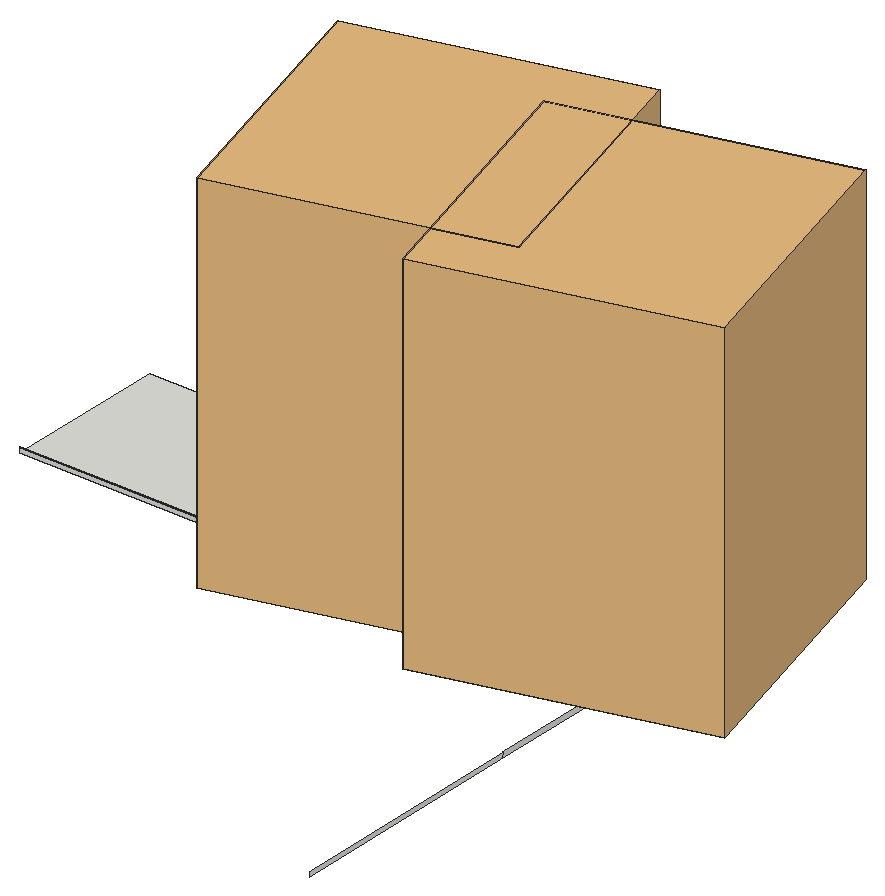
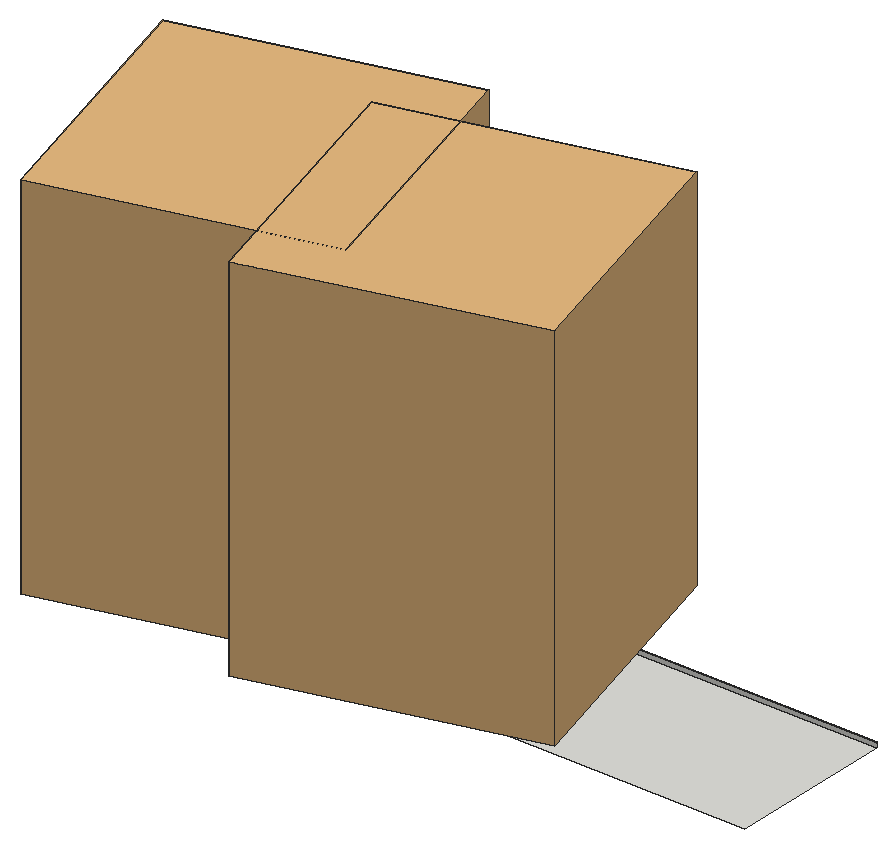
# SketchUp Ruby script. Lengths in inches.
U = 1.inch
M = Sketchup.active_model
def pt(a) = Geom::Point3d.new(a.map { |v| v * U })
def face(e, loops, mat)
  f = e.add_face(loops[0].map { |a| pt(a) })
  loops[1..].each { |l| e.add_face(l.map { |a| pt(a) }).erase! }
  f.material = f.back_material = mat if mat
  f
end
# faces: each face lists its corners as indices into pts; further lists are holes
def faces(e, pts, list, mat = nil) = list.each { |f| face(e, (f[0].is_a?(Array) ? f : [f]).map { |l| l.map { |i| pts[i] } }, mat) }
# xy, xz, yz: faces in a plane at the given z, y or x. An outline is a flat list of corners, or four numbers for a rectangle; further outlines are holes
def ring(l) = l.size == 4 ? [[l[0], l[1]], [l[2], l[1]], [l[2], l[3]], [l[0], l[3]]] : l.each_slice(2).to_a
def flat(e, list, mat, &to3) = list.each { |f| face(e, (f[0].is_a?(Array) ? f : [f]).map { |l| ring(l).map { |u, v| to3.(u, v) } }, mat) }
def xy(e, z, list, mat = nil) = flat(e, list, mat) { |x, y| [x, y, z] }
def xz(e, y, list, mat = nil) = flat(e, list, mat) { |x, z| [x, y, z] }
def yz(e, x, list, mat = nil) = flat(e, list, mat) { |y, z| [x, y, z] }
def lines(e, pts, list) = list.each { |a, b| e.add_line(pt(pts[a]), pt(pts[b])) }
# prism: a flat outline (further loops are holes) pulled along v
def prism(e, loops, v, mat = nil)
  f = face(e, loops, mat); d = Geom::Vector3d.new(v.map { |x| x * U })
  f.pushpull(f.normal.samedirection?(d) ? d.length : -d.length)
end
def box(e, o, s, mat = nil) = prism(e, [[o, [o[0] + s[0], o[1], o[2]], [o[0] + s[0], o[1] + s[1], o[2]], [o[0], o[1] + s[1], o[2]]]], [0, 0, s[2]], mat)
def at(x, y, z, deg = 0) = Geom::Transformation.translation(pt([x, y, z])) * Geom::Transformation.rotation(ORIGIN, Z_AXIS, deg.degrees)
def axes(o, x, y, z) = Geom::Transformation.new([*x, 0, *y, 0, *z, 0, *pt(o).to_a, 1])
def part(name) = M.definitions.add(name)
# library, detail: a bought-in or finely detailed component or shape, given as its bounding box
def library(name, o, s) = part(name).tap { |d| box(d.entities, o, s) }
def detail(e, o, s) = box(e.add_group.entities, o, s)
def put(e, d, t, mat = nil) = e.add_instance(d, t).tap { |i| i.material = mat if mat }
def group(e, t, mat = nil) = e.add_group.tap { |g| g.transformation = t; g.material = mat if mat }.entities
root = M.entities
M.materials.add("Material82").color = [68, 110, 58]
M.materials.add("Material83").color = [48, 90, 38]
M.materials.add("Material84").color = [68, 110, 48]
M.materials.add("Material85").color = [48, 90, 48]
M.materials.add("Material86").color = [58, 110, 58]
M.materials.add("Material87").color = [58, 90, 38]
M.materials.add("Material88").color = [68, 100, 58]
M.materials.add("Material89").color = [48, 100, 38]
c1 = part("grass00")
p = [[-0.6875,0.15,0],[-0.56,0.08,5.52],[-0.04,0.03,2.76],[0.48,-0.02,0],[0.35,-0.02,5.52],[-0.1,-0.14,5.52],
  [-0.12,0.65,8.37],[-0.42,0.65,8.37]]
faces(c1.entities,p,[[0,1,2,3],[3,2,4],[1,5,2],[5,4,2],[1,6,5],[4,5,6],[7,6,1]])
c2 = part("Group16\#1")
put(c2.entities,c1,axes([1.44,-0.61,-0.01],[0.05352,0.12609,0],[-0.10704,0.04543,0.07239],[0.06664,-0.02828,0.11628]),"Material85")
put(c2.entities,c1,axes([0.76,-0.15,-0.01],[0.04676,0.24062,0],[-0.23162,0.04501,0.06642],[0.0652,-0.01267,0.23595]),"Material82")
put(c2.entities,c1,axes([0.79,0.01,-0.01],[-0.00606,0.34651,0],[-0.34381,-0.00602,0.0432],[0.04319,0.00076,0.34386]))
put(c2.entities,c1,axes([1,0.23,-0.01],[-0.07192,0.31144,0],[-0.28722,-0.06632,0.1236],[0.12043,0.02781,0.29478]),"Material84")
put(c2.entities,c1,axes([1.66,0.77,-0.01],[-0.13828,0.29651,0],[-0.21551,-0.1005,0.22471],[0.20365,0.09498,0.23779]),"Material89")
put(c2.entities,c1,axes([0.6875,0.52,-0.01],[-0.18126,0.24051,0],[-0.22746,-0.17142,0.09788],[0.07817,0.05891,0.28481]),"Material84")
put(c2.entities,c1,axes([0.68,0.78,-0.01],[-0.215,0.18688,0],[-0.12385,-0.14248,0.21334],[0.13995,0.16101,0.18878]),"Material82")
put(c2.entities,c1,axes([0.56,1,-0.01],[-0.13756,0.07624,0],[-0.06159,-0.11112,0.0927],[0.04494,0.08108,0.12705]),"Material84")
put(c2.entities,c1,axes([0.2,0.64,-0.01],[-0.23729,0.07254,0],[-0.05711,-0.18681,0.153],[0.04473,0.14632,0.19535]),"Material89")
put(c2.entities,c1,axes([0.0625,0.72,-0.01],[-0.28874,0.02525,0],[-0.02179,-0.24916,0.14647],[0.01276,0.14591,0.25012]),"Material82")
put(c2.entities,c1,axes([-0.08,0.62,-0.01],[-0.34089,-0.04187,0],[0.03255,-0.26504,0.216],[-0.02633,0.21439,0.26703]),"Material89")
put(c2.entities,c1,axes([-0.34,0.98,-0.01],[-0.14314,-0.0493,0],[0.04397,-0.12769,0.06843],[-0.02228,0.0647,0.13505]),"Material89")
put(c2.entities,c1,axes([-0.87,1.45,-0.01],[-0.23488,-0.14114,0],[0.13761,-0.22901,0.06087],[-0.03135,0.05217,0.26717]))
put(c2.entities,c1,axes([-0.72,0.77,-0.01],[-0.14208,-0.13251,0],[0.07209,-0.0773,0.16301],[-0.11118,0.11922,0.1057]),"Material89")
put(c2.entities,c1,axes([-0.62,0.43,-0.01],[-0.14845,-0.21203,0],[0.18654,-0.13061,0.12304],[-0.10079,0.07057,0.22772]),"Material82")
put(c2.entities,c1,axes([-0.68,0.29,-0.01],[-0.13639,-0.32136,0],[0.31723,-0.13464,0.05579],[-0.05136,0.0218,0.34462]),"Material83")
put(c2.entities,c1,axes([-0.64,0.125,-0.01],[-0.0458,-0.23569,0],[0.22124,-0.043,0.08276],[-0.08124,0.01579,0.22538]),"Material86")
put(c2.entities,c1,axes([-1.6,-0.03,-0.01],[0.00576,-0.32897,0],[0.27526,0.00482,0.18018],[-0.18015,-0.00315,0.2753]),"Material84")
put(c2.entities,c1,axes([-1.36,-0.31,-0.01],[0.05718,-0.24765,0],[0.18172,0.04196,0.17267],[-0.16825,-0.03885,0.1865]),"Material89")
put(c2.entities,c1,axes([-1.54,-0.72,-0.01],[0.06537,-0.14017,0],[0.13555,0.06321,0.03939],[-0.0357,-0.01665,0.14956]))
put(c2.entities,c1,axes([-1.19,-0.9,-0.01],[0.09597,-0.12735,0],[0.11214,0.08451,0.07557],[-0.06035,-0.04548,0.14042]),"Material88")
put(c2.entities,c1,axes([-0.47,-0.54,-0.01],[0.11588,-0.10072,0],[0.0618,0.0711,0.12124],[-0.07953,-0.0915,0.0942]))
put(c2.entities,c1,axes([-0.47,-0.84,-0.01],[0.11927,-0.0661,0],[0.06603,0.11913,0.00646],[-0.00313,-0.00565,0.13621]),"Material84")
put(c2.entities,c1,axes([-0.38,-1.24,-0.01],[0.28037,-0.08571,0],[0.0618,0.20215,0.20315],[-0.05939,-0.19428,0.21139]),"Material88")
put(c2.entities,c1,axes([-0.06,-0.66,-0.01],[0.22719,-0.01987,0],[0.01247,0.14255,0.17758],[-0.01547,-0.17691,0.1431]),"Material87")
put(c2.entities,c1,axes([0.11,-0.89,-0.01],[0.14882,0.01828,0],[-0.01058,0.08611,0.12229],[0.01491,-0.12138,0.08676]),"Material85")
put(c2.entities,c1,axes([0.25,-0.72,-0.01],[0.20481,0.07053,0],[-0.06206,0.18022,0.10291],[0.03351,-0.0973,0.1906]),"Material85")
put(c2.entities,c1,axes([0.85,-1.42,-0.01],[0.16481,0.09904,0],[-0.09472,0.15762,0.05616],[0.02893,-0.04814,0.18389]),"Material84")
put(c2.entities,c1,axes([1.01,-1.09,-0.01],[0.21858,0.20385,0],[-0.17495,0.1876,0.15339],[0.10462,-0.11218,0.25652]),"Material89")
put(c2.entities,c1,axes([1.01,-0.71,-0.01],[0.08733,0.12473,0],[-0.06445,0.04512,0.13037],[0.1068,-0.07477,0.07867]),"Material85")
c3 = part("Group15\#1")
put(c3.entities,c2,at(0,0,0))
c4 = part("3darcstudiotree_grass00\#1")
put(c4.entities,c3,at(0,0,0))
c5 = library("Palm tree",[-4.09,-4.52,0],[193.52,193.51,258.93])
c6 = part("Palm+Tree")
put(c6.entities,c5,at(25.51,-21.81,0,15))
c7 = library("Group\#612",[0,0,0],[32.91,53.52,103.45])
xy(root,-42.1875,[[1674.99,273.41,2096.97,387.84]])
xz(root,273.41,[[1674.99,-42.1875,2096.97,-42.1875,2096.97,-38.61,1897.28,-38.61,1897.28,-39.125,1674.99,-39.125],[1674.99,-38.61,2096.97,-38.1875]])
yz(root,2096.97,[[1.59,-42.1875,172.28,-39.1875],[172.28,-42.1875,273.41,-38.61],[273.41,-42.1875,387.84,-34.17]])
put(root,c4,axes([1856.99,323.88,-34.17],[-2.27595,1.46975,0],[-3.85308,-0.92798,-0.0342],[-0.14118,-0.034,1.63693]))
put(root,c4,axes([1856.66,307.49,-34.17],[3.38368,1.04745,0],[-2.27938,1.14521,-0.02005],[-0.08327,0.04184,1.86077]))
put(root,c4,axes([1858.71,335.1875,-34.17],[0.01113,-1.45353,0],[4.54919,0.00542,-0.03692],[0.17089,0.0002,1.57831]))
put(root,c4,axes([1859.04,313.29,-34.17],[-1.2969,-1.20265,0],[3.80092,-0.63749,-0.01791],[0.10113,-0.01696,1.89984]))
put(root,c4,axes([1859.15,291.65,-34.17],[0.25593,-1.38573,0],[3.33259,0.09573,-0.00937],[0.07232,0.00208,1.93766]))
put(root,c4,axes([1859.03,287.07,-34.17],[-3.13946,0.49629,0],[-1.50487,-1.48058,-0.04281],[-0.09532,-0.09378,1.81418]))
put(root,c4,axes([1858.93,329.8125,-34.17],[3.11316,-1.08854,0],[2.76667,1.23063,-0.03392],[0.0954,0.04244,1.32537]))
put(root,c4,axes([1860.03,298.21,-34.17],[-3.90762,0.14516,0],[-0.37668,-1.57704,-0.0202],[-0.01231,-0.05153,1.95637]))
put(root,c4,axes([1860.17,339.86,-34.17],[-1.14276,-1.73672,0],[3.49011,-0.35717,-0.03225],[0.18285,-0.01871,1.58326]))
put(root,c4,axes([1858.89,282.42,-34.17],[3.63772,-0.04618,0],[0.1059,1.29755,-0.04101],[0.00733,0.08987,1.37186]))
put(root,c4,axes([1858.96,337.85,-34.17],[0.13497,1.53866,0],[-3.75353,0.05121,-0.02489],[-0.17047,0.00233,1.9295]))
put(root,c4,axes([1859.52,333.37,-34.17],[-2.50392,0.92561,0],[-3.00944,-1.26617,-0.02311],[-0.06646,-0.02796,1.38694]))
put(root,c4,axes([1860.67,326.64,-34.17],[-4.13167,0.24366,0],[-0.69238,-1.82599,-0.06496],[-0.05165,-0.1362,1.88637]))
put(root,c4,axes([1859.86,309.54,-34.17],[-1.70819,1.11812,0],[-3.96876,-0.943,-0.04504],[-0.21667,-0.05148,1.9506]))
put(root,c4,axes([1860.05,318.65,-34.17],[3.79912,-1.05543,0],[2.19489,1.22878,-0.03692],[0.13668,0.07652,1.83631]))
put(root,c4,axes([1859.92,284.9,-34.17],[3.28657,0.21022,0],[-0.53923,1.31117,-0.01255],[-0.01302,0.03166,1.63564]))
put(root,c4,axes([1860.52,324.84,-34.17],[-2.37455,1.29783,0],[-2.73236,-0.77752,-0.00844],[-0.03827,-0.01089,1.41311]))
put(root,c4,axes([1859.85,315.9,-34.17],[2.3712,1.21069,0],[-3.58151,1.09097,-0.04605],[-0.15475,0.04714,1.44046]))
put(root,c4,axes([1861.08,301.02,-34.17],[1.66455,-1.14728,0],[3.31311,0.74761,-0.04415],[0.26641,0.06012,1.98924]))
put(root,c4,axes([1862.18,331.24,-34.17],[-0.63027,-1.58552,0],[4.65732,-0.28794,-0.06318],[0.24644,-0.01524,1.39517]))
put(root,c4,axes([1860.64,302.46,-34.17],[2.52471,1.58546,0],[-3.52346,0.87265,-0.052],[-0.25077,0.06211,1.7759]))
put(root,c4,axes([1861.42,323.25,-34.17],[3.33412,-1.28398,0],[2.96352,1.19685,-0.04175],[0.14903,0.06019,1.62422]))
put(root,c4,axes([1860.82,319.77,-34.17],[3.98735,0.11869,0],[-0.3473,1.81468,-0.00004],[-0.00002,0.00009,1.93334]))
put(root,c4,axes([1862.46,294.22,-34.17],[-2.08457,-1.53905,0],[3.84719,-0.81044,-0.05822],[0.30315,-0.06386,1.92982]))
put(root,c4,axes([1861.59,311.12,-34.17],[0.24653,1.78059,0],[-4.18646,0.09015,-0.05861],[-0.36644,0.00789,1.96776]))
put(root,c4,axes([1861.1,305.77,-34.17],[4.09909,0.70116,0],[-1.55013,1.40946,-0.01845],[-0.03388,0.03081,1.34771]))
put(root,c4,axes([1861.13,281.39,-34.17],[1.95248,1.61036,0],[-3.842,0.72449,-0.01048],[-0.04175,0.00787,1.40926]))
put(root,c4,axes([1861.45,296.15,-34.17],[3.93599,0.37319,0],[-1.10472,1.81211,-0.03506],[-0.03066,0.05029,1.32515]))
put(root,c4,axes([1862.1,289.81,-34.17],[3.76504,-0.34797,0],[1.07827,1.81452,-0.02268],[0.0226,0.03802,1.5468]))
put(root,c4,axes([1862.1,306.82,-34.17],[-0.03028,1.81071,0],[-4.52004,-0.01176,-0.01347],[-0.05788,-0.00015,1.45625]))
put(root,c4,axes([1864.3125,288.28,-34.17],[2.88127,-0.83898,0],[2.47269,1.32072,-0.02283],[0.06307,0.03369,1.4512]))
put(root,c4,axes([1865.23,293.27,-34.17],[-1.69688,-1.72936,0],[4.23511,-0.64631,-0.05475],[0.2829,-0.04317,1.88574]))
put(root,c4,axes([1864.3125,285.39,-34.17],[3.22121,-0.88629,0],[2.07064,1.17047,-0.00731],[0.02777,0.0157,1.80073]))
put(root,c4,axes([1865.44,335.42,-34.17],[-1.90792,-1.42621,0],[3.47826,-0.72369,-0.03938],[0.16408,-0.03414,1.38871]))
put(root,c4,axes([1864.51,322.01,-34.17],[3.56261,-0.94567,0],[1.87037,1.0959,-0.0013],[0.00431,0.00253,1.49257]))
put(root,c4,axes([1864.41,296.77,-34.17],[-1.05565,1.36177,0],[-3.91341,-0.47183,-0.0271],[-0.14616,-0.01762,1.72974]))
put(root,c4,axes([1865.7,289.4375,-34.17],[-4.0685,0.50795,0],[-1.17773,-1.46714,-0.03323],[-0.06082,-0.07576,1.77353]))
put(root,c4,axes([1864.76,282.8,-34.17],[4.25936,0.17724,0],[-0.36955,1.38123,-0.03171],[-0.02162,0.08082,1.71518]))
put(root,c4,axes([1866.37,299.0625,-34.17],[0.20903,-1.7077,0],[3.89534,0.07416,-0.00402],[0.01821,0.00035,1.3243]))
put(root,c4,axes([1866.48,305.18,-34.17],[-3.49989,-0.62042,0],[1.34924,-1.18377,-0.02079],[0.0557,-0.04887,1.61237]))
put(root,c4,axes([1865.74,307.34,-34.17],[-2.24971,1.27376,0],[-2.901,-0.79689,-0.01437],[-0.08541,-0.02346,1.91898]))
put(root,c4,axes([1866.64,329.74,-34.17],[-2.13915,-1.27276,0],[3.26215,-0.85272,-0.05028],[0.27845,-0.07279,1.94898]))
put(root,c4,axes([1865.51,333.7,-34.17],[4.02195,-0.32221,0],[0.68718,1.33408,-0.00331],[0.00405,0.00786,1.58887]))
put(root,c4,axes([1865,320,-34.17],[4.32701,0.55712,0],[-1.36775,1.65217,-0.00124],[-0.00192,0.00232,1.65228]))
put(root,c4,axes([1866.2,327.39,-34.17],[-1.63539,1.16071,0],[-3.40916,-0.74706,-0.05151],[-0.29339,-0.06429,1.90487]))
put(root,c4,axes([1865.4,324.48,-34.17],[1.01762,1.37596,0],[-4.26505,0.49058,-0.00405],[-0.01582,0.00182,1.35389]))
put(root,c4,axes([1867.69,316.36,-34.17],[-3.3697,-1.02042,0],[2.44227,-1.25434,-0.00705],[0.02625,-0.01348,1.8369]))
put(root,c4,axes([1866.83,317.9375,-34.17],[2.02024,-1.18426,0],[3.76291,0.99837,-0.06298],[0.20491,0.05437,1.33293]))
put(root,c4,axes([1866.05,281.31,-34.17],[4.3094,-0.16311,0],[0.42718,1.75528,-0.01064],[0.00539,0.02213,1.77558]))
put(root,c4,axes([1867.82,331.57,-34.17],[-2.95002,-1.42448,0],[3.56758,-1.14909,-0.03335],[0.13906,-0.04479,1.85855]))
put(root,c4,axes([1867.24,312.33,-34.17],[0.35372,-1.85816,0],[4.64402,0.13749,-0.06273],[0.35272,0.01044,1.9684]))
put(root,c4,axes([1866.83,291.29,-34.17],[-1.74852,1.13217,0],[-3.21789,-0.77293,-0.03041],[-0.12145,-0.02917,1.3205]))
put(root,c4,axes([1868.16,310.09,-34.17],[-1.80602,-1.23313,0],[3.1704,-0.72217,-0.00817],[0.04009,-0.00913,1.55447]))
put(root,c4,axes([1866.43,338.45,-34.17],[3.63959,0.40285,0],[-0.8944,1.25675,-0.00495],[-0.00749,0.01053,1.38942]))
put(root,c4,axes([1867.4,313.01,-34.17],[3.72507,-0.62439,0],[1.73357,1.60854,-0.00549],[0.00931,0.00864,1.44062]))
put(root,c4,axes([1867.39,301.21,-34.17],[3.99736,-0.43263,0],[1.22188,1.75587,-0.05143],[0.05673,0.08152,1.44218]))
put(root,c4,axes([1867.36,303.03,-34.17],[-0.70731,1.48216,0],[-4.42453,-0.32839,-0.01956],[-0.1033,-0.00767,1.8138]))
put(root,c4,axes([1869.84,298.91,-34.17],[-4.33089,0.41445,0],[-1.11243,-1.80796,-0.06662],[-0.06204,-0.10083,1.39642]))
put(root,c4,axes([1870.72,289.05,-34.17],[-3.26976,-0.5137,0],[1.67175,-1.65498,-0.00121],[0.00254,-0.00252,1.92636]))
put(root,c4,axes([1869.96,333.375,-34.17],[1.4091,-1.17417,0],[3.00858,0.56155,-0.04441],[0.31581,0.05895,1.96303]))
put(root,c4,axes([1870.7,329.09,-34.17],[-0.33318,-1.39627,0],[3.47077,-0.12881,-0.04952],[0.2452,-0.0091,1.29958]))
put(root,c4,axes([1870.81,324.74,-34.17],[-3.53744,1.16554,0],[-2.5606,-1.20869,-0.03098],[-0.10582,-0.04995,1.59479]))
put(root,c4,axes([1871.42,337.18,-34.17],[-3.84526,-0.22431,0],[0.50015,-1.33348,-0.00812],[0.00644,-0.01718,1.3892]))
put(root,c4,axes([1870.94,319.86,-34.17],[-3.00421,0.76942,0],[-2.15411,-1.30812,-0.04277],[-0.14646,-0.08894,1.86401]))
put(root,c4,axes([1870.4,291.51,-34.17],[-0.58592,1.57945,0],[-3.44253,-0.19862,-0.02144],[-0.15876,-0.00916,1.9513]))
put(root,c4,axes([1870.91,312.34,-34.17],[-3.04736,0.88871,0],[-2.40783,-1.28411,-0.01371],[-0.03527,-0.01881,1.31321]))
put(root,c4,axes([1870.41,331.78,-34.17],[3.34176,-0.01383,0],[0.04057,1.52455,-0.01029],[0.00052,0.01945,1.389]))
put(root,c4,axes([1871.53,296.11,-34.17],[1.49416,-1.17809,0],[3.55261,0.70077,-0.01805],[0.08589,0.01694,1.58457]))
put(root,c4,axes([1870.65,318.32,-34.17],[3.91979,-0.74164,0],[1.60866,1.32236,-0.04597],[0.11253,0.0925,1.57738]))
put(root,c4,axes([1870.83,315.58,-34.17],[-2.1963,1.32957,0],[-3.96988,-1.01993,-0.00953],[-0.0332,-0.00853,1.47621]))
put(root,c4,axes([1872.09,335.79,-34.17],[0.96851,-1.36822,0],[3.89034,0.4283,-0.00232],[0.01298,0.00143,1.76107]))
put(root,c4,axes([1871.09,322.77,-34.17],[3.27047,-0.2692,0],[0.72961,1.37861,-0.04941],[0.05481,0.10356,1.4533]))
put(root,c4,axes([1872.31,305.79,-34.17],[2.10515,-1.21949,0],[3.30844,0.88826,-0.01892],[0.09087,0.0244,1.74337]))
put(root,c4,axes([1872.19,284.625,-34.17],[-2.16702,1.28274,0],[-3.03597,-0.79769,-0.03773],[-0.16249,-0.04269,1.41517]))
put(root,c4,axes([1871.42,326.65,-34.17],[4.03817,0.43694,0],[-1.08149,1.5545,-0.02738],[-0.04454,0.06402,1.88342]))
put(root,c4,axes([1871.97,312.99,-34.17],[4.33985,-0.71517,0],[1.81915,1.7169,-0.05614],[0.0962,0.09079,1.57175]))
put(root,c4,axes([1872.99,301.33,-34.17],[1.94166,-1.68054,0],[3.68889,0.66287,-0.02827],[0.1643,0.02952,1.94019]))
put(root,c4,axes([1872.3,307.22,-34.17],[0.75441,1.71197,0],[-3.26624,0.22386,-0.03272],[-0.2394,0.01641,1.8454]))
put(root,c4,axes([1872.03,309.46,-34.17],[2.94946,0.97112,0],[-2.79078,1.31828,-0.05497],[-0.191,0.09022,1.76958]))
put(root,c4,axes([1872.01,302.05,-34.17],[2.19107,1.06462,0],[-2.74426,0.87841,-0.00448],[-0.02021,0.00647,1.5389]))
put(root,c4,axes([1873.16,294.37,-34.17],[2.33071,-1.20912,0],[3.74929,1.12403,-0.05929],[0.20074,0.06018,1.50135]))
put(root,c4,axes([1872.91,283.1,-34.17],[-0.50717,1.45325,0],[-4.1597,-0.22578,-0.0385],[-0.18859,-0.01024,1.55608]))
put(root,c4,axes([1873.3,287.78,-34.17],[4.27397,-0.60338,0],[1.4489,1.5962,-0.05713],[0.08848,0.09748,1.48067]))
put(root,c4,axes([1875.34,326.3,-34.17],[-2.9256,-1.47399,0],[3.63184,-1.12114,-0.01534],[0.06015,-0.01857,1.72134]))
put(root,c4,axes([1875.125,311.77,-34.17],[-4.1987,0.12334,0],[-0.25997,-1.37638,-0.0204],[-0.0079,-0.04182,1.3669]))
put(root,c4,axes([1875.5,330.98,-34.17],[-4.00085,-0.57986,0],[1.27846,-1.37193,-0.00277],[0.00474,-0.00509,1.38049]))
put(root,c4,axes([1876.02,314.24,-34.17],[-3.39001,-0.81782,0],[2.4179,-1.55881,-0.03935],[0.08518,-0.05492,1.44076]))
put(root,c4,axes([1875.33,287.1,-34.17],[3.84648,-0.75898,0],[1.52103,1.1989,-0.01525],[0.0428,0.03373,1.59832]))
put(root,c4,axes([1875.97,320.33,-34.17],[2.20697,-0.9726,0],[2.75858,0.97355,-0.01984],[0.09708,0.03426,1.82222]))
put(root,c4,axes([1875.79,315.36,-34.17],[0.68368,1.71904,0],[-3.38759,0.20954,-0.03929],[-0.29518,0.01826,1.95437]))
put(root,c4,axes([1877.26,322.4375,-34.17],[-2.04632,-1.05436,0],[3.10393,-0.93693,-0.02737],[0.09658,-0.02915,1.30175]))
put(root,c4,axes([1876.18,308.98,-34.17],[-0.28903,1.73584,0],[-3.34699,-0.08668,-0.03425],[-0.21957,-0.00569,1.61497]))
put(root,c4,axes([1877.02,329.46,-34.17],[1.71259,-1.30416,0],[3.53393,0.72176,-0.01075],[0.04765,0.00973,1.48923]))
put(root,c4,axes([1877.3,295.62,-34.17],[-3.772,0.03773,0],[-0.10384,-1.61464,-0.00196],[-0.00024,-0.00377,1.49745]))
put(root,c4,axes([1876.64,290.01,-34.17],[-2.36342,1.1502,0],[-3.36153,-1.07427,-0.04128],[-0.15124,-0.04833,1.52936]))
put(root,c4,axes([1876.21,294.41,-34.17],[4.05183,0.05747,0],[-0.14664,1.60785,-0.02702],[-0.00634,0.06949,1.99535]))
put(root,c4,axes([1877.12,338.34,-34.17],[2.29885,-0.96399,0],[2.83055,1.04983,-0.02136],[0.08662,0.03213,1.62144]))
put(root,c4,axes([1877.85,292.19,-34.17],[-4.17405,-0.19289,0],[0.40333,-1.35747,-0.00847],[0.00693,-0.02334,1.82708]))
put(root,c4,axes([1876.8,318.61,-34.17],[1.65421,1.20964,0],[-3.07102,0.65317,-0.03445],[-0.21317,0.04534,1.83855]))
put(root,c4,axes([1878.49,286.15,-34.17],[-2.90823,-0.76432,0],[2.41266,-1.42777,-0.04785],[0.14851,-0.08788,1.82518]))
put(root,c4,axes([1877.52,305.75,-34.17],[-1.04428,1.44728,0],[-3.25699,-0.36551,-0.00052],[-0.00331,-0.00037,1.67384]))
put(root,c4,axes([1877.65,306.83,-34.17],[3.83018,0.17914,0],[-0.49889,1.65896,-0.05841],[-0.02825,0.09394,1.30397]))
put(root,c4,axes([1879.17,299.99,-34.17],[-3.60335,-0.2844,0],[0.69529,-1.3701,-0.00178],[0.00231,-0.00455,1.75352]))
put(root,c4,axes([1878.625,324.37,-34.17],[-2.93874,0.89671,0],[-2.33959,-1.1925,-0.04163],[-0.12402,-0.06321,1.39503]))
put(root,c4,axes([1877.76,333.02,-34.17],[2.61631,0.861,0],[-2.17217,1.02658,-0.00812],[-0.03307,0.01563,1.6158]))
put(root,c4,axes([1877.73,298.75,-34.17],[2.19518,1.25426,0],[-3.21279,0.87453,-0.02215],[-0.10628,0.02893,1.70619]))
put(root,c4,axes([1878.4,282.39,-34.17],[0.43339,1.54675,0],[-3.36238,0.14653,-0.03685],[-0.25104,0.01094,1.73767]))
put(root,c4,axes([1878.57,339.96,-34.17],[3.63873,-0.8009,0],[1.86273,1.31624,-0.03495],[0.11311,0.07993,1.90256]))
put(root,c4,axes([1878.03,334.85,-34.17],[3.82301,1.06562,0],[-2.5922,1.44638,-0.0169],[-0.04207,0.02347,1.45184]))
put(root,c4,axes([1878.97,302.78,-34.17],[3.73956,-0.25134,0],[0.58802,1.36068,-0.03176],[0.03776,0.08738,1.85682]))
put(root,c4,axes([1880.84,295.76,-34.17],[-2.3605,-1.50274,0],[2.8114,-0.68684,-0.00146],[0.00663,-0.00162,1.32424]))
put(root,c4,axes([1880.8,290.26,-34.17],[3.76532,-0.82989,0],[2.11238,1.49062,-0.04605],[0.09606,0.06778,1.38783]))
put(root,c4,axes([1882.0625,287.23,-34.17],[-2.75712,-0.97177,0],[2.36987,-1.04575,-0.04195],[0.16334,-0.07208,1.55746]))
put(root,c4,axes([1880.63,333.26,-34.17],[1.13904,1.65719,0],[-4.07352,0.43546,-0.03421],[-0.20227,0.02162,1.93796]))
put(root,c4,axes([1882.64,303.49,-34.17],[-1.0442,-1.68413,0],[4.42012,-0.42624,-0.03172],[0.12352,-0.01191,1.36741]))
put(root,c4,axes([1882.79,283.2,-34.17],[-2.93582,-0.70247,0],[2.08855,-1.35755,-0.00574],[0.01328,-0.00863,1.3472]))
put(root,c4,axes([1882.81,312.27,-34.17],[-2.87675,-1.09055,0],[2.6601,-1.09136,-0.02949],[0.13969,-0.05731,1.96656]))
put(root,c4,axes([1882.96,317.73,-34.17],[-2.96111,-1.38906,0],[2.74036,-0.90856,-0.02964],[0.13819,-0.04582,1.63454]))
put(root,c4,axes([1881.36,301.13,-34.17],[2.75422,1.28702,0],[-2.68657,0.89417,-0.05003],[-0.26479,0.08813,1.82479]))
put(root,c4,axes([1881.53,307.34,-34.17],[2.36808,1.36159,0],[-2.95794,0.80011,-0.03781],[-0.20263,0.05481,1.74723]))
put(root,c4,axes([1881.58,335.56,-34.17],[4.47082,0.11069,0],[-0.26321,1.65346,-0.04601],[-0.01202,0.07548,1.31249]))
put(root,c4,axes([1882.23,316.08,-34.17],[-2.49032,1.32428,0],[-3.19574,-0.93467,-0.0152],[-0.05407,-0.01581,1.3203]))
put(root,c4,axes([1881.68,308.59,-34.17],[1.04539,1.48143,0],[-4.29845,0.47176,-0.02844],[-0.1492,0.01637,1.82107]))
put(root,c4,axes([1882.45,329.1,-34.17],[-2.32252,1.56487,0],[-3.68383,-0.85034,-0.03733],[-0.14959,-0.03453,1.48568]))
put(root,c4,axes([1881.84,323.96,-34.17],[2.07418,1.09295,0],[-3.13936,0.92662,-0.0157],[-0.06877,0.0203,1.60759]))
put(root,c4,axes([1882.54,304.39,-34.17],[3.63146,-0.94763,0],[2.16895,1.29272,-0.03005],[0.10609,0.06323,1.88475]))
put(root,c4,axes([1881.9,339.45,-34.17],[4.62364,0.41674,0],[-0.83657,1.44354,-0.00333],[-0.00361,0.00623,1.36941]))
put(root,c4,axes([1882.13,314.51,-34.17],[0.90968,1.754,0],[-3.81846,0.30801,-0.01369],[-0.06439,0.00519,1.40267]))
put(root,c4,axes([1882.73,285.43,-34.17],[0.278,1.64734,0],[-3.85699,0.10123,-0.01024],[-0.06423,0.00169,1.82096]))
put(root,c4,axes([1883.22,321.67,-34.17],[-1.2304,1.69187,0],[-3.83777,-0.43408,-0.02925],[-0.12783,-0.01446,1.36051]))
put(root,c4,axes([1882.89,327.29,-34.17],[2.50159,1.07866,0],[-2.96417,1.06917,-0.03451],[-0.16033,0.05783,1.89576]))
put(root,c4,axes([1883.03,331.67,-34.17],[3.85299,0.72056,0],[-1.4234,1.18377,-0.0026],[-0.00811,0.00675,1.81639]))
put(root,c4,axes([1884.59,294.17,-34.17],[-3.94572,0.20967,0],[-0.54102,-1.58348,-0.01091],[-0.00895,-0.02619,1.8656]))
put(root,c4,axes([1883.23,291.15,-34.17],[4.67805,0.10708,0],[-0.2535,1.72242,-0.0212],[-0.00736,0.05004,1.96575]))
put(root,c4,axes([1883.52,319.91,-34.17],[3.89819,0.51903,0],[-1.48599,1.73579,-0.0473],[-0.0826,0.09649,1.90097]))
put(root,c4,axes([1883.59,338.21,-34.17],[3.72345,0.43237,0],[-1.05501,1.41306,-0.01058],[-0.0164,0.02196,1.53588]))
put(root,c4,axes([1883.75,298.4,-34.17],[3.62609,0.38691,0],[-0.94095,1.37154,-0.04799],[-0.07441,0.10847,1.60328]))
put(root,c4,axes([1886.85,287.81,-34.17],[-2.74827,-0.90606,0],[2.5057,-1.18207,-0.04185],[0.15974,-0.07536,1.7425]))
put(root,c4,axes([1887.125,319.83,-34.17],[-2.21298,-1.13198,0],[3.27865,-0.99688,-0.03514],[0.15829,-0.04813,1.76492]))
put(root,c4,axes([1887.0625,331.16,-34.17],[1.56077,-1.21628,0],[3.51485,0.70149,-0.00728],[0.02929,0.00585,1.33141]))
put(root,c4,axes([1886.55,333.29,-34.17],[-1.38329,1.54062,0],[-3.20389,-0.44741,-0.04758],[-0.27737,-0.03873,1.57537]))
put(root,c4,axes([1887.6,291.96,-34.17],[-4.11808,-0.53305,0],[1.24091,-1.491,-0.0393],[0.07027,-0.08443,1.71017]))
put(root,c4,axes([1887.17,322.96,-34.17],[-3.99092,0.85507,0],[-1.6879,-1.22527,-0.00649],[-0.01661,-0.01206,1.42064]))
put(root,c4,axes([1886.52,335.81,-34.17],[-0.13254,1.67215,0],[-3.60359,-0.04442,-0.04056],[-0.20717,-0.00255,1.38085]))
put(root,c4,axes([1887.37,302.03,-34.17],[-1.8566,1.22673,0],[-3.23788,-0.76215,-0.0186],[-0.08298,-0.01953,1.46845]))
put(root,c4,axes([1887.55,312.94,-34.17],[3.63516,-0.37062,0],[1.04175,1.58916,-0.04398],[0.06662,0.10163,1.88821]))
put(root,c4,axes([1887.5,283.5,-34.17],[4.38242,0.53414,0],[-1.34963,1.72221,-0.04987],[-0.06942,0.08859,1.61513]))
put(root,c6,at(1831.89,232.43,-34.17))
put(root,c7,axes([1999.58,235.4,-34.17],[1.13014,0.75656,0],[-0.75656,1.13014,0],[0,0,1.36]))
put(root,c6,at(1977.26,232.43,-34.17))
